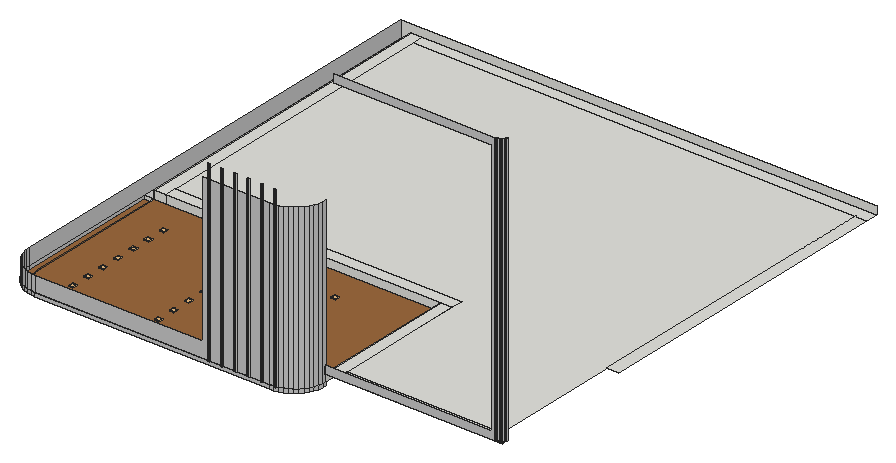
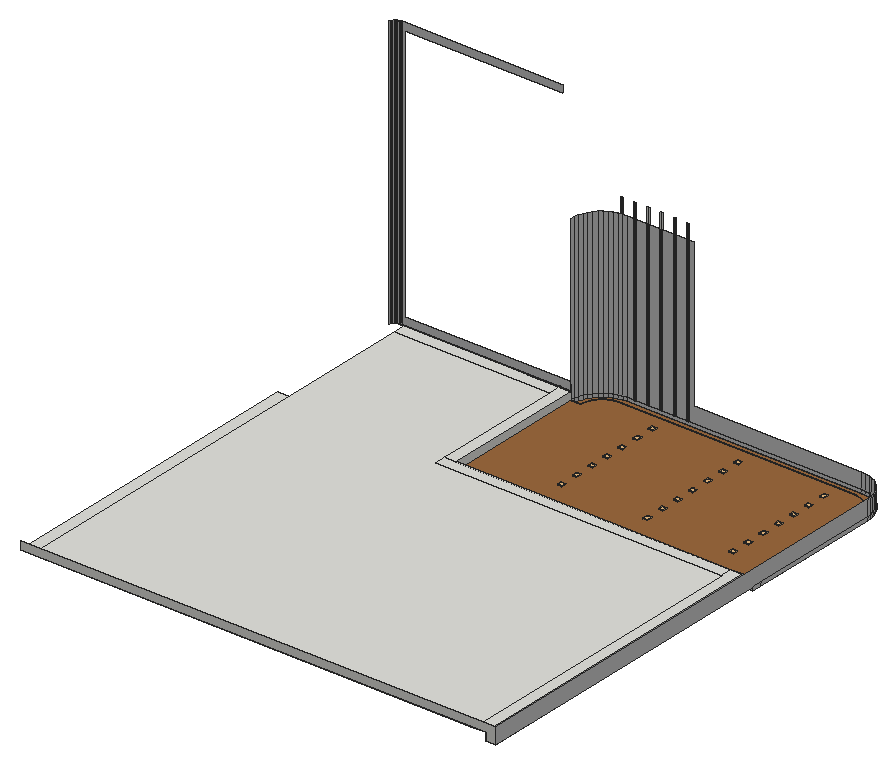
# SketchUp Ruby script. Lengths in inches.
U = 1.inch
M = Sketchup.active_model
def pt(a) = Geom::Point3d.new(a.map { |v| v * U })
def face(e, loops, mat)
  f = e.add_face(loops[0].map { |a| pt(a) })
  loops[1..].each { |l| e.add_face(l.map { |a| pt(a) }).erase! }
  f.material = f.back_material = mat if mat
  f
end
# faces: each face lists its corners as indices into pts; further lists are holes
def faces(e, pts, list, mat = nil) = list.each { |f| face(e, (f[0].is_a?(Array) ? f : [f]).map { |l| l.map { |i| pts[i] } }, mat) }
# xy, xz, yz: faces in a plane at the given z, y or x. An outline is a flat list of corners, or four numbers for a rectangle; further outlines are holes
def ring(l) = l.size == 4 ? [[l[0], l[1]], [l[2], l[1]], [l[2], l[3]], [l[0], l[3]]] : l.each_slice(2).to_a
def flat(e, list, mat, &to3) = list.each { |f| face(e, (f[0].is_a?(Array) ? f : [f]).map { |l| ring(l).map { |u, v| to3.(u, v) } }, mat) }
def xy(e, z, list, mat = nil) = flat(e, list, mat) { |x, y| [x, y, z] }
def xz(e, y, list, mat = nil) = flat(e, list, mat) { |x, z| [x, y, z] }
def yz(e, x, list, mat = nil) = flat(e, list, mat) { |y, z| [x, y, z] }
def lines(e, pts, list) = list.each { |a, b| e.add_line(pt(pts[a]), pt(pts[b])) }
# prism: a flat outline (further loops are holes) pulled along v
def prism(e, loops, v, mat = nil)
  f = face(e, loops, mat); d = Geom::Vector3d.new(v.map { |x| x * U })
  f.pushpull(f.normal.samedirection?(d) ? d.length : -d.length)
end
def box(e, o, s, mat = nil) = prism(e, [[o, [o[0] + s[0], o[1], o[2]], [o[0] + s[0], o[1] + s[1], o[2]], [o[0], o[1] + s[1], o[2]]]], [0, 0, s[2]], mat)
def at(x, y, z, deg = 0) = Geom::Transformation.translation(pt([x, y, z])) * Geom::Transformation.rotation(ORIGIN, Z_AXIS, deg.degrees)
def axes(o, x, y, z) = Geom::Transformation.new([*x, 0, *y, 0, *z, 0, *pt(o).to_a, 1])
def part(name) = M.definitions.add(name)
# library, detail: a bought-in or finely detailed component or shape, given as its bounding box
def library(name, o, s) = part(name).tap { |d| box(d.entities, o, s) }
def detail(e, o, s) = box(e.add_group.entities, o, s)
def put(e, d, t, mat = nil) = e.add_instance(d, t).tap { |i| i.material = mat if mat }
def group(e, t, mat = nil) = e.add_group.tap { |g| g.transformation = t; g.material = mat if mat }.entities
root = M.entities
M.materials.add("[Cladding Stucco White]").color = [200, 200, 200]
M.materials.add("[Color M01]").color = [226, 226, 226]
M.materials.add("[Wood Floor]").color = [155, 105, 61]
c1 = library("Tlon Light 650 Ceiling 152 007",[-12.8,-12.8,-3.78],[25.6,25.6,3.58])
xy(root,111.125,[[24,0.91,21.1,1.1,18.01,1.72,15.03,2.73,12.2,4.125,9.58,5.875,7.21,7.96,5.125,10.33,3.375,12.95,1.98,15.78,0.97,18.76,0.35,21.85,0.16,24.75,0.16,128.51,0.1875,128.51,0.1875,136.0625,7.9375,136.0625,7.85,128.46,7.85,128.4,7.875,128.375,7.875,25.25,8.03,22.86,8.45,20.77,9.14,18.74,10.08,16.82,11.27,15.04,12.68,13.43,14.29,12.02,16.07,10.83,17.99,9.89,20.02,9.2,22.11,8.78,24.5,8.625,205.625,8.625,208.01,8.78,210.11,9.2,212.14,9.89,214.05,10.83,215.83,12.02,217.44,13.43,218.85,15.04,220.04,16.82,220.99,18.74,221.68,20.77,222.09,22.86,222.14,22.86,222.28,25.0625,229.94,25.0625,229.73,21.86,229.77,21.85,229.16,18.76,228.14,15.78,226.75,12.95,225,10.33,222.92,7.96,220.55,5.875,217.93,4.125,215.1,2.73,212.11,1.72,209.02,1.1,206.125,0.91]],"[Wood Floor]")
xy(root,114,[[157.86,0.51,159.39,0.91],[168.11,0.51,169.64,0.91],[178.36,0.51,179.89,0.91],[188.61,0.51,190.14,0.91],[198.86,0.51,200.39,0.91],
  [209.11,0.51,210.64,0.91]])
xy(root,114,[[0.25,136.0625,7.875,385]],"[Cladding Stucco White]")
xy(root,114,[[24.5,8.625,22.11,8.78,20.02,9.2,17.99,9.89,16.07,10.83,14.29,12.02,12.68,13.43,11.27,15.04,10.08,16.82,9.14,18.74,8.45,20.77,8.03,22.86,7.875,25.25,7.875,128.375,7.85,128.4,7.85,128.46,7.9375,136,229.875,136,229.875,25.0625,222.28,25.0625,222.14,22.86,222.09,22.86,221.68,20.77,220.99,18.74,220.04,16.82,218.85,15.04,217.44,13.43,215.83,12.02,214.05,10.83,212.14,9.89,210.11,9.2,208.01,8.78,205.625,8.625]],"[Wood Floor]")
xy(root,120,[[229.875,24,238.875,25],[238.875,24,263.375,25],[263.375,24,358.875,25],[358.875,24,367.875,25],[229.875,25,238.875,136],
  [238.875,25,358.875,34],[238.875,34,238.875,145,16.875,145,16.875,376,358.875,376,358.875,34],[7.875,136,16.875,385],[16.875,136,238.875,145],[358.875,136,367.875,376],
  [16.875,376,367.875,385]])
xy(root,120.1875,[[361.5625,24,367.875,24,367.875,28.62,367.57,27.92,367.19,27.27,366.75,26.65,366.24,26.09,365.68,25.58,365.07,25.14,364.41,24.76,363.72,24.45,362.99,24.22,362.25,24.07]])
xy(root,251.12,[[209.11,0.53,210.64,0.93]])
xz(root,0.91,[[24,111.125,206.125,114]],"[Cladding Stucco White]")
xz(root,0.9375,[[24.25,111.125,205.88,114]],"[Cladding Stucco White]")
xz(root,1,[[24.25,114,205.875,114,205.875,240,154.02,240,154.02,126,24.25,126]],"[Cladding Stucco White]")
xz(root,8.6,[[24.25,111.125,205.87,114]])
xz(root,8.625,[[24.5,111.125,205.625,114]],"[Wood Floor]")
xz(root,24,[[229.875,120,367.875,120,367.875,120.1875,361.5625,120.1875,361.5625,330,236.52,330,236.52,324,358.875,324,358.875,126,229.875,126]],"[Cladding Stucco White]")
xz(root,25.0625,[[222.28,111.125,229.94,114]])
xz(root,136,[[7.875,114,16.875,120],[16.875,114,229.875,120]])
xz(root,136.0625,[[0.1875,111.125,7.9375,114]])
xz(root,385,[[0.25,114,0.25,126,367.875,126,367.875,120,7.875,120,7.875,114]])
yz(root,0.16,[[24.75,111.125,128.51,114]],"[Cladding Stucco White]")
yz(root,0.1875,[[25,111.125,136.0625,114]],"[Cladding Stucco White]")
yz(root,0.25,[[25,114,385,126]],"[Cladding Stucco White]")
yz(root,7.85,[[25,111.125,128.46,114]])
yz(root,7.875,[[136,114,385,120]])
yz(root,7.875,[[25.25,111.125,128.375,114]],"[Wood Floor]")
yz(root,157.86,[[0.51,114,0.53,251.12,0.93,251.12,0.91,114]])
yz(root,159.39,[[0.51,114,0.91,114,0.93,251.12,0.53,251.12]])
yz(root,168.11,[[0.51,114,0.53,251.12,0.93,251.12,0.91,114]])
yz(root,169.64,[[0.51,114,0.91,114,0.93,251.12,0.53,251.12]])
yz(root,178.36,[[0.51,114,0.53,251.12,0.93,251.12,0.91,114]])
yz(root,179.89,[[0.51,114,0.91,114,0.93,251.12,0.53,251.12]])
yz(root,188.61,[[0.51,114,0.53,251.12,0.93,251.12,0.91,114]])
yz(root,190.14,[[0.51,114,0.91,114,0.93,251.12,0.53,251.12]])
yz(root,198.86,[[0.51,114,0.53,251.12,0.93,251.12,0.91,114]])
yz(root,200.39,[[0.51,114,0.91,114,0.93,251.12,0.53,251.12]])
yz(root,209.11,[[0.51,114,0.53,251.12,0.93,251.12,0.91,114]])
yz(root,210.64,[[0.51,114,0.91,114,0.93,251.12,0.53,251.12]])
yz(root,229.875,[[25,114,136,120],[24,120,25,126]])
p = [[21.11,1.14,114],[21.11,1.14,111.125],[24,0.95,111.125],[24.25,0.9375,111.125],[24.25,0.9375,114],[24,0.95,114],
  [24,0.91,111.125],[24,0.91,114],[21.1,1.1,114],[21.1,1.1,111.125],[205.88,0.9375,114],[205.88,0.9375,111.125],
  [209.02,1.14,111.125],[209.02,1.14,114],[206.125,0.95,114],[209.02,1.1,111.125],[209.02,1.1,114],[206.125,0.91,114],
  [206.125,0.91,111.125],[18.02,1.76,114],[18.02,1.76,111.125],[18.01,1.72,114],[18.01,1.72,111.125],[212.1,1.76,111.125],
  [212.1,1.76,114],[212.11,1.72,111.125],[212.11,1.72,114],[15.03,2.73,114],[15.03,2.73,111.125],[215.1,2.73,111.125],
  [215.1,2.73,114],[15.04,2.77,114],[15.04,2.77,111.125],[215.08,2.77,111.125],[215.08,2.77,114],[12.2,4.125,114],
  [12.2,4.125,111.125],[217.93,4.125,111.125],[217.93,4.125,114],[12.22,4.16,114],[12.22,4.16,111.125],[217.91,4.16,111.125],
  [217.91,4.16,114],[9.58,5.875,114],[9.58,5.875,111.125],[220.55,5.875,111.125],[220.55,5.875,114],[9.6,5.91,114],
  [9.6,5.91,111.125],[220.52,5.91,111.125],[220.52,5.91,114],[7.24,7.99,114],[7.24,7.99,111.125],[7.21,7.96,114],
  [7.21,7.96,111.125],[222.89,7.99,111.125],[222.89,7.99,114],[222.92,7.96,111.125],[222.92,7.96,114],[5.125,10.33,114],
  [5.125,10.33,111.125],[5.16,10.35,114],[5.16,10.35,111.125],[224.97,10.35,111.125],[224.97,10.35,114],[225,10.33,111.125],
  [225,10.33,114],[24.25,8.6,114],[24.25,8.6,111.125],[22.11,8.74,111.125],[22.11,8.74,114],[22.11,8.78,111.125],
  [22.11,8.78,114],[24.5,8.625,114],[24.5,8.625,111.125],[205.625,8.625,111.125],[205.625,8.625,114],[208.01,8.78,114],
  [208.01,8.78,111.125],[208.02,8.74,114],[208.02,8.74,111.125],[205.87,8.6,111.125],[205.87,8.6,114],[20.01,9.16,111.125],
  [20.01,9.16,114],[210.12,9.16,114],[210.12,9.16,111.125],[20.02,9.2,111.125],[20.02,9.2,114],[210.11,9.2,114],
  [210.11,9.2,111.125],[17.97,9.85,111.125],[17.97,9.85,114],[17.99,9.89,111.125],[17.99,9.89,114],[212.15,9.85,114],
  [212.15,9.85,111.125],[212.14,9.89,114],[212.14,9.89,111.125],[16.05,10.8,111.125],[16.05,10.8,114],[214.08,10.8,114],
  [214.08,10.8,111.125],[16.07,10.83,111.125],[16.07,10.83,114],[214.05,10.83,114],[214.05,10.83,111.125],[3.375,12.95,114],
  [3.375,12.95,111.125],[226.75,12.95,111.125],[226.75,12.95,114],[3.41,12.97,114],[3.41,12.97,111.125],[226.71,12.97,111.125],
  [226.71,12.97,114],[14.27,11.99,111.125],[14.27,11.99,114],[14.29,12.02,111.125],[14.29,12.02,114],[215.86,11.99,114],
  [215.86,11.99,111.125],[215.83,12.02,114],[215.83,12.02,111.125],[12.65,13.4,111.125],[12.65,13.4,114],[12.68,13.43,111.125],
  [12.68,13.43,114],[217.44,13.43,114],[217.44,13.43,111.125],[217.47,13.4,114],[217.47,13.4,111.125],[1.98,15.78,114],
  [1.98,15.78,111.125],[228.14,15.78,111.125],[228.14,15.78,114],[2.02,15.79,114],[2.02,15.79,111.125],[228.11,15.79,111.125],
  [228.11,15.79,114],[11.24,15.02,111.125],[11.24,15.02,114],[11.27,15.04,111.125],[11.27,15.04,114],[218.85,15.04,114],
  [218.85,15.04,111.125],[218.89,15.02,114],[218.89,15.02,111.125],[10.05,16.8,111.125],[10.05,16.8,114],[10.08,16.82,111.125],
  [10.08,16.82,114],[220.08,16.8,114],[220.08,16.8,111.125],[220.04,16.82,114],[220.04,16.82,111.125],[1.01,18.77,114],
  [1.01,18.77,111.125],[0.97,18.76,114],[0.97,18.76,111.125],[229.12,18.77,111.125],[229.12,18.77,114],[229.16,18.76,111.125],
  [229.16,18.76,114],[9.1,18.72,111.125],[9.1,18.72,114],[9.14,18.74,111.125],[9.14,18.74,114],[220.99,18.74,114],
  [220.99,18.74,111.125],[221.03,18.72,114],[221.03,18.72,111.125],[8.41,20.76,111.125],[8.41,20.76,114],[8.45,20.77,111.125],
  [8.45,20.77,114],[221.72,20.76,114],[221.72,20.76,111.125],[221.68,20.77,114],[221.68,20.77,111.125],[0.39,21.86,114],
  [0.39,21.86,111.125],[0.35,21.85,114],[0.35,21.85,111.125],[229.73,21.86,111.125],[229.73,21.86,114],[229.77,21.85,111.125],
  [229.77,21.85,114],[7.99,22.86,111.125],[7.99,22.86,114],[8.03,22.86,111.125],[8.03,22.86,114],[222.14,22.86,114],
  [222.14,22.86,111.125],[222.09,22.86,114],[222.09,22.86,111.125],[0.1875,25,114],[0.1875,25,111.125],[0.16,24.75,114],
  [0.16,24.75,111.125],[229.94,25.0625,111.125],[229.94,25.0625,114],[7.85,25,111.125],[7.85,25,114],[7.875,25.25,111.125],
  [7.875,25.25,114],[222.28,25.0625,114],[222.28,25.0625,111.125],[7.85,128.46,114],[7.85,128.46,111.125],[7.9375,136.0625,111.125],
  [7.9375,136.0625,114],[7.9375,136,114],[157.86,0.53,251.12],[157.86,0.51,114],[159.39,0.51,114],[159.39,0.53,251.12],
  [168.11,0.53,251.12],[168.11,0.51,114],[169.64,0.51,114],[169.64,0.53,251.12],[178.36,0.53,251.12],[178.36,0.51,114],
  [179.89,0.51,114],[179.89,0.53,251.12],[188.61,0.53,251.12],[188.61,0.51,114],[190.14,0.51,114],[190.14,0.53,251.12],
  [198.86,0.53,251.12],[198.86,0.51,114],[200.39,0.51,114],[200.39,0.53,251.12],[209.11,0.53,251.12],[209.11,0.51,114],
  [210.64,0.51,114],[210.64,0.53,251.12],[209.11,0.91,114],[209.11,0.93,251.12],[210.64,0.93,251.12],[210.64,0.91,114],
  [24.21,1,126],[21.12,1.21,126],[21.12,1.21,114],[24.25,1,114],[24.25,1,126],[209.01,1.21,114],
  [209.01,1.21,240],[205.875,1,240],[205.875,1,114],[18.04,1.82,126],[18.04,1.82,114],[212.09,1.82,114],
  [212.09,1.82,240],[15.07,2.83,126],[15.07,2.83,114],[215.06,2.83,114],[215.06,2.83,240],[12.25,4.22,126],
  [12.25,4.22,114],[217.875,4.22,114],[217.875,4.22,240],[9.64,5.96,126],[9.64,5.96,114],[220.49,5.96,114],
  [220.49,5.96,240],[7.28,8.03,126],[7.28,8.03,114],[222.85,8.03,114],[222.85,8.03,240],[5.21,10.39,126],
  [5.21,10.39,114],[224.92,10.39,114],[224.92,10.39,240],[3.47,13,126],[3.47,13,114],[226.66,13,114],
  [226.66,13,240],[2.08,15.82,126],[2.08,15.82,114],[228.05,15.82,114],[228.05,15.82,240],[1.07,18.79,126],
  [1.07,18.79,114],[229.06,18.79,114],[229.06,18.79,240],[0.46,21.87,126],[0.46,21.87,114],[229.67,21.87,114],
  [229.67,21.87,240],[0.25,25,126],[0.25,25,114],[229.875,25,120],[229.875,25,126],[229.875,25,127.5625],
  [229.875,25,128.63],[229.875,25,130.125],[229.875,25,131.2],[229.875,25,132.6875],[229.875,25,133.76],[229.875,25,135.25],
  [229.875,25,136.32],[229.875,25,137.8125],[229.875,25,138.88],[229.875,25,140.375],[229.875,25,141.45],[229.875,25,142.75],
  [229.875,25,143.82],[229.875,25,145.0625],[229.875,25,146.13],[229.875,25,147.5],[229.875,25,148.57],[229.875,25,150.0625],
  [229.875,25,151.13],[229.875,25,152.5625],[229.875,25,153.63],[229.875,25,155.0625],[229.875,25,156.13],[229.875,25,157.5625],
  [229.875,25,158.63],[229.875,25,160.0625],[229.875,25,161.13],[229.875,25,162.5625],[229.875,25,163.63],[229.875,25,165.0625],
  [229.875,25,166.13],[229.875,25,167.5625],[229.875,25,168.63],[229.875,25,170.0625],[229.875,25,171.13],[229.875,25,172.5625],
  [229.875,25,173.63],[229.875,25,175.0625],[229.875,25,176.13],[229.875,25,177.75],[229.875,25,178.82],[229.875,25,180.4375],
  [229.875,25,181.51],[229.875,25,183.125],[229.875,25,184.2],[229.875,25,185.8125],[229.875,25,186.88],[229.875,25,188.5],
  [229.875,25,189.57],[229.875,25,191.1875],[229.875,25,192.26],[229.875,25,193.875],[229.875,25,194.95],[229.875,25,196.5625],
  [229.875,25,197.63],[229.875,25,199.25],[229.875,25,200.32],[229.875,25,201.9375],[229.875,25,203.01],[229.875,25,204.625],
  [229.875,25,205.7],[229.875,25,207.3125],[229.875,25,208.38],[229.875,25,210],[229.875,25,211.07],[229.875,25,212.6875],
  [229.875,25,213.76],[229.875,25,215.375],[229.875,25,216.45],[229.875,25,217.9375],[229.875,25,219.01],[229.875,25,220.875],
  [229.875,25,221.95],[229.875,25,223.8125],[229.875,25,224.88],[229.875,25,226.75],[229.875,25,227.82],[229.875,25,229.6875],
  [229.875,25,230.76],[229.875,25,232.375],[229.875,25,233.45],[229.875,25,235.0625],[229.875,25,236.13],[229.875,25,237.75],
  [229.875,25,238.82],[229.875,25,240],[229.875,25,114],[362.25,24.07,330],[361.5625,24,330],[361.5625,24,120.1875],
  [362.25,24.07,120.1875],[362.99,24.22,330],[362.99,24.22,120.1875],[363.72,24.45,330],[363.72,24.45,120.1875],[364.41,24.76,330],
  [364.41,24.76,120.1875],[365.07,25.14,330],[365.07,25.14,120.1875],[365.68,25.58,330],[365.68,25.58,120.1875],[366.24,26.09,330],
  [366.24,26.09,120.1875],[366.75,26.65,330],[366.75,26.65,120.1875],[367.19,27.27,330],[367.19,27.27,120.1875],[367.57,27.92,330],
  [367.57,27.92,120.1875],[367.875,28.62,330],[367.875,28.62,120.1875],[229.76,23.17,119.17],[220.89,0.91,114],[219.36,0.91,114]]
faces(root,p,[[0,1,2,3,4,5],[6,7,8,9],[10,11,12,13,14],[15,16,17,18],[19,20,1,0],[9,8,21,22],[13,12,23,24],[25,26,16,15],
  [22,21,27,28],[29,30,26,25],[31,32,20,19],[24,23,33,34],[28,27,35,36],[37,38,30,29],[39,40,32,31],[34,33,41,42],
  [36,35,43,44],[45,46,38,37],[47,48,40,39],[42,41,49,50],[51,52,48,47],[44,43,53,54],[50,49,55,56],[57,58,46,45],
  [54,53,59,60],[61,62,52,51],[56,55,63,64],[65,66,58,57],[60,59,107,108],[109,110,66,65],[111,112,62,61],[64,63,113,114],
  [108,107,131,132],[133,134,110,109],[135,136,112,111],[114,113,137,138],[155,156,136,135],[132,131,157,158],[138,137,159,160],[161,162,134,133],
  [179,180,156,155],[158,157,181,182],[160,159,183,184],[185,186,162,161],[195,196,180,179],[182,181,197,198],[184,183,199,200],[240,241,242,243,244],
  [245,246,247,248],[241,249,250,242],[251,252,246,245],[249,253,254,250],[255,256,252,251],[253,257,258,254],[259,260,256,255],[257,261,262,258],
  [263,264,260,259],[261,265,266,262],[267,268,264,263],[265,269,270,266],[271,272,268,267],[269,273,274,270],[275,276,272,271],[273,277,278,274],
  [279,280,276,275],[277,281,282,278],[283,284,280,279],[281,285,286,282],[287,288,284,283],[285,289,290,286],[291,292,293,294,295,296,297,298,299,300,301,302,303,304,305,306,307,308,309,310,311,312,313,314,315,316,317,318,319,320,321,322,323,324,325,326,327,328,329,330,331,332,333,334,335,336,337,338,339,340,341,342,343,344,345,346,347,348,349,350,351,352,353,354,355,356,357,358,359,360,361,362,363,364,365,366,367,368,369,370,371,372,373,374,375,376,377,378,379,288,287,380],[381,382,383,384],
  [385,381,384,386],[387,385,386,388],[389,387,388,390],[391,389,390,392],[393,391,392,394],[395,393,394,396],[397,395,396,398],[399,397,398,400],
  [401,399,400,402],[403,401,402,404]],"[Cladding Stucco White]")
faces(root,p,[[67,68,69,70],[79,80,81,82],[70,69,83,84],[85,86,80,79],[84,83,91,92],[95,96,86,85],[92,91,99,100],[101,102,96,95],
  [100,99,115,116],[119,120,102,101],[116,115,123,124],[129,130,120,119],[124,123,139,140],[145,146,130,129],[140,139,147,148],[151,152,146,145],
  [148,147,163,164],[169,170,152,151],[164,163,171,172],[175,176,170,169],[172,171,187,188],[191,192,176,175],[188,187,201,202],[205,206,192,191],
  [207,208,209,210,211],[236,237,238,239]])
faces(root,p,[[71,72,73,74],[75,76,77,78],[87,88,72,71],[78,77,89,90],[93,94,88,87],[90,89,97,98],[103,104,94,93],[98,97,105,106],
  [117,118,104,103],[106,105,121,122],[125,126,118,117],[122,121,127,128],[141,142,126,125],[128,127,143,144],[149,150,142,141],[144,143,153,154],
  [165,166,150,149],[154,153,167,168],[173,174,166,165],[168,167,177,178],[189,190,174,173],[178,177,193,194],[203,204,190,189]],"[Wood Floor]")
faces(root,p,[[212,213,214,215],[216,217,218,219],[220,221,222,223],[224,225,226,227],[228,229,230,231],[232,233,234,235]],"[Color M01]")
lines(root,p,[[405,291],[406,407]])
put(root,c1,axes([36.6,80.24,114.43],[0.14,0,0],[0,0.14,0],[0,0,0.14]))
put(root,c1,axes([36.6,94.86,114.43],[0.14,0,0],[0,0.14,0],[0,0,0.14]))
put(root,c1,axes([36.6,109.49,114.43],[0.14,0,0],[0,0.14,0],[0,0,0.14]))
put(root,c1,axes([36.6,50.99,114.43],[0.14,0,0],[0,0.14,0],[0,0,0.14]))
put(root,c1,axes([36.6,36.36,114.43],[0.14,0,0],[0,0.14,0],[0,0,0.14]))
put(root,c1,axes([36.6,21.74,114.43],[0.14,0,0],[0,0.14,0],[0,0,0.14]))
put(root,c1,axes([36.6,65.61,114.43],[0.14,0,0],[0,0.14,0],[0,0,0.14]))
put(root,c1,axes([102.98,109.49,114.43],[0.14,0,0],[0,0.14,0],[0,0,0.14]))
put(root,c1,axes([102.98,21.74,114.43],[0.14,0,0],[0,0.14,0],[0,0,0.14]))
put(root,c1,axes([102.98,65.61,114.43],[0.14,0,0],[0,0.14,0],[0,0,0.14]))
put(root,c1,axes([102.98,50.99,114.43],[0.14,0,0],[0,0.14,0],[0,0,0.14]))
put(root,c1,axes([102.98,36.36,114.43],[0.14,0,0],[0,0.14,0],[0,0,0.14]))
put(root,c1,axes([102.98,80.24,114.43],[0.14,0,0],[0,0.14,0],[0,0,0.14]))
put(root,c1,axes([102.98,94.86,114.43],[0.14,0,0],[0,0.14,0],[0,0,0.14]))
put(root,c1,axes([169.35,109.49,114.43],[0.14,0,0],[0,0.14,0],[0,0,0.14]))
put(root,c1,axes([169.35,21.74,114.43],[0.14,0,0],[0,0.14,0],[0,0,0.14]))
put(root,c1,axes([169.35,65.61,114.43],[0.14,0,0],[0,0.14,0],[0,0,0.14]))
put(root,c1,axes([169.35,50.99,114.43],[0.14,0,0],[0,0.14,0],[0,0,0.14]))
put(root,c1,axes([169.35,36.36,114.43],[0.14,0,0],[0,0.14,0],[0,0,0.14]))
put(root,c1,axes([169.35,80.24,114.43],[0.14,0,0],[0,0.14,0],[0,0,0.14]))
put(root,c1,axes([169.35,94.86,114.43],[0.14,0,0],[0,0.14,0],[0,0,0.14]))
